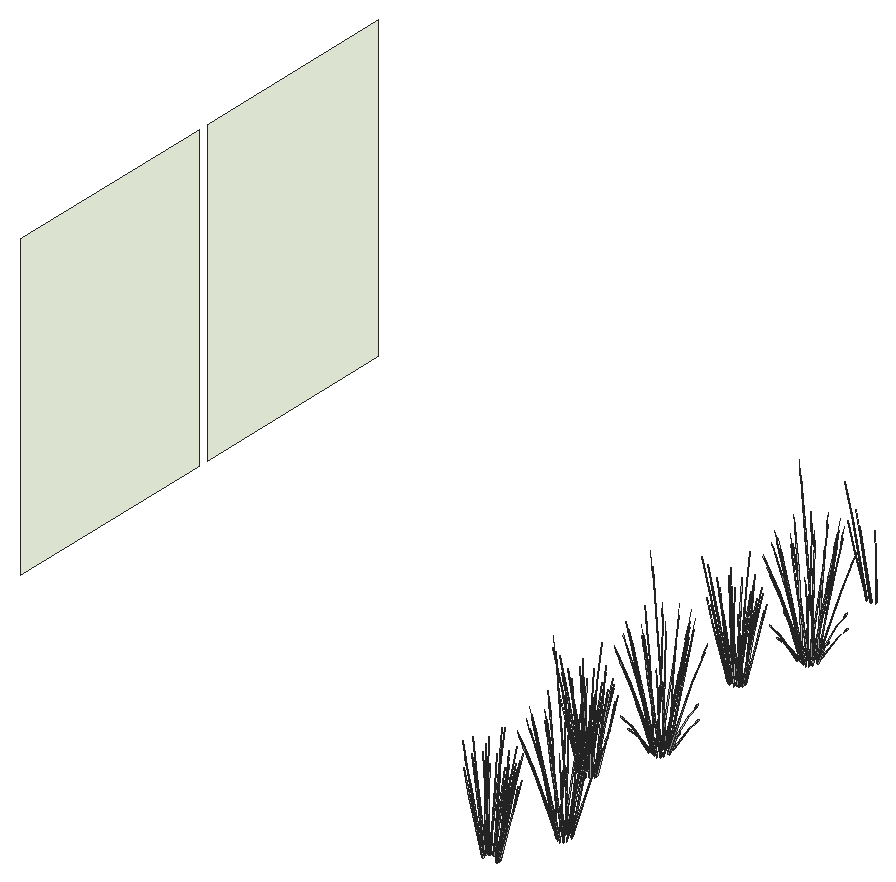
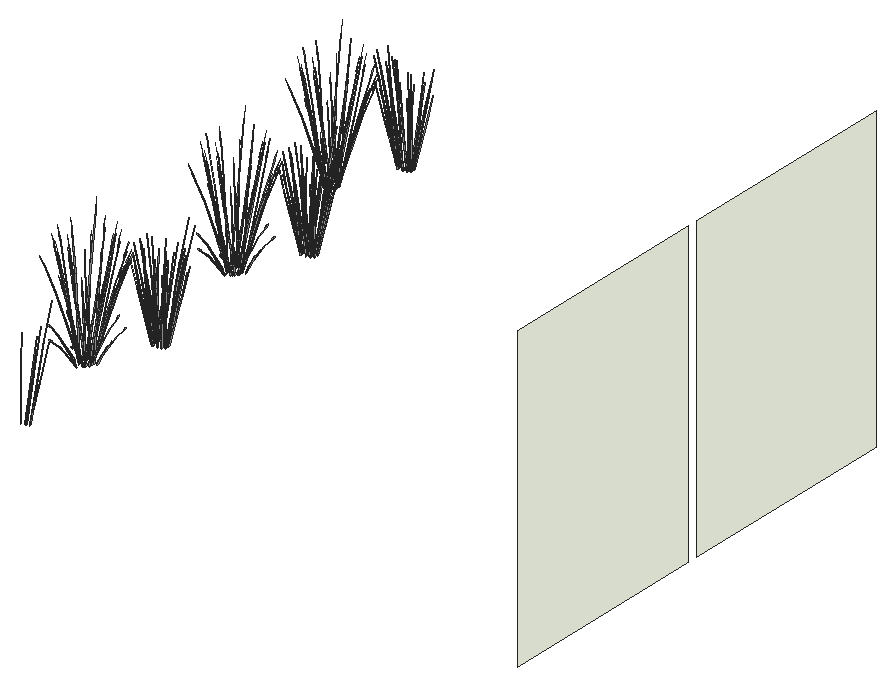
# SketchUp Ruby script. Lengths in inches.
U = 1.inch
M = Sketchup.active_model
def pt(a) = Geom::Point3d.new(a.map { |v| v * U })
def face(e, loops, mat)
  f = e.add_face(loops[0].map { |a| pt(a) })
  loops[1..].each { |l| e.add_face(l.map { |a| pt(a) }).erase! }
  f.material = f.back_material = mat if mat
  f
end
# faces: each face lists its corners as indices into pts; further lists are holes
def faces(e, pts, list, mat = nil) = list.each { |f| face(e, (f[0].is_a?(Array) ? f : [f]).map { |l| l.map { |i| pts[i] } }, mat) }
# xy, xz, yz: faces in a plane at the given z, y or x. An outline is a flat list of corners, or four numbers for a rectangle; further outlines are holes
def ring(l) = l.size == 4 ? [[l[0], l[1]], [l[2], l[1]], [l[2], l[3]], [l[0], l[3]]] : l.each_slice(2).to_a
def flat(e, list, mat, &to3) = list.each { |f| face(e, (f[0].is_a?(Array) ? f : [f]).map { |l| ring(l).map { |u, v| to3.(u, v) } }, mat) }
def xy(e, z, list, mat = nil) = flat(e, list, mat) { |x, y| [x, y, z] }
def xz(e, y, list, mat = nil) = flat(e, list, mat) { |x, z| [x, y, z] }
def yz(e, x, list, mat = nil) = flat(e, list, mat) { |y, z| [x, y, z] }
def lines(e, pts, list) = list.each { |a, b| e.add_line(pt(pts[a]), pt(pts[b])) }
# prism: a flat outline (further loops are holes) pulled along v
def prism(e, loops, v, mat = nil)
  f = face(e, loops, mat); d = Geom::Vector3d.new(v.map { |x| x * U })
  f.pushpull(f.normal.samedirection?(d) ? d.length : -d.length)
end
def box(e, o, s, mat = nil) = prism(e, [[o, [o[0] + s[0], o[1], o[2]], [o[0] + s[0], o[1] + s[1], o[2]], [o[0], o[1] + s[1], o[2]]]], [0, 0, s[2]], mat)
def at(x, y, z, deg = 0) = Geom::Transformation.translation(pt([x, y, z])) * Geom::Transformation.rotation(ORIGIN, Z_AXIS, deg.degrees)
def axes(o, x, y, z) = Geom::Transformation.new([*x, 0, *y, 0, *z, 0, *pt(o).to_a, 1])
def part(name) = M.definitions.add(name)
# library, detail: a bought-in or finely detailed component or shape, given as its bounding box
def library(name, o, s) = part(name).tap { |d| box(d.entities, o, s) }
def detail(e, o, s) = box(e.add_group.entities, o, s)
def put(e, d, t, mat = nil) = e.add_instance(d, t).tap { |i| i.material = mat if mat }
def group(e, t, mat = nil) = e.add_group.tap { |g| g.transformation = t; g.material = mat if mat }.entities
root = M.entities
M.materials.add("Glass_Basic_1").color = [156, 186, 90]
M.materials["Glass_Basic_1"].alpha = 0.25
M.materials.add("LightPink_Translucent").color = [175, 214, 192]
M.materials["LightPink_Translucent"].alpha = 0.75
c1 = part("blade")
p = [[2.15,0.21,22],[0,0.17,0],[0.09,0.45,0],[2.18,0.31,22],[2.29,0.31,22],[0.38,0.45,0],
  [2.48,0.24,33],[2.49,0.24,33],[2.48,0.22,33]]
faces(c1.entities,p,[[0,1,2,3],[4,5,2,3],[6,3,4,7],[8,0,3,6]])
c2 = part("blade with seeds\#1")
put(c2.entities,c1,at(0,0,0))
c3 = part("seeds")
p = [[0.3,-0.1,1.38],[-0.01,-0.03,1.59],[-0.01,-0.03,0.03],[0.14,-0.07,-0.07],[0.29,-0.03,3],[0.15,0.01,3.11]]
faces(c3.entities,p,[[0,1,2,3],[1,0,4,5]],"LightPink_Translucent")
c4 = part("blade with seeds")
put(c4.entities,c1,at(0,0,0))
put(c4.entities,c3,axes([2.4,0.25,30.99],[1.5799,-0.05474,1.17369],[-0.12525,1.92788,0.29478],[-0.07173,-0.02425,1.56792]))
yz(root,330,[[388.5,141,453,228],[456,141,517.5,228]],"Glass_Basic_1")
put(root,c2,axes([495.49,353.2,140.96],[-0.43273,0.05446,0.29052],[-0.11427,-0.31131,-0.37506],[0.12401,-0.08362,0.71765]))
put(root,c2,axes([495.79,353.08,140.7],[0.12329,0.35069,0.39379],[-0.48364,0.06086,0.3247],[0.14254,-0.08248,0.81485]))
put(root,c2,axes([495.88,353.15,140.69],[0.34128,0.16025,0.05275],[-0.1987,0.22821,0.41527],[0.10942,-0.07378,0.63322]))
put(root,c2,axes([492.04,352.71,140.96],[0.28286,0.23857,0.29052],[-0.32298,0.22584,-0.37506],[-0.1641,-0.03436,0.71765]))
put(root,c2,axes([495.56,353.94,140.96],[-0.41315,-0.1063,0.29052],[0.1205,-0.31012,-0.37506],[0.16634,-0.02844,0.71765]))
put(root,c2,axes([491.24,353.375,140.7],[0.14045,-0.34743,0.39379],[0.46175,0.1188,0.3247],[-0.18159,0.02088,0.81485]))
put(root,c2,axes([491.2,353.28,140.69],[-0.18259,-0.25981,0.05275],[0.33295,-0.12717,0.41527],[-0.14677,0.02509,0.63322]))
put(root,c2,axes([495.93,354.04,140.69],[0.18259,0.25981,0.05275],[-0.33295,0.12717,0.41527],[0.14677,-0.02509,0.63322]))
put(root,c2,axes([495.9,353.94,140.7],[-0.14045,0.34743,0.39379],[-0.46175,-0.1188,0.3247],[0.18159,-0.02088,0.81485]))
put(root,c2,axes([491.57,353.38,140.96],[0.41315,0.1063,0.29052],[-0.1205,0.31012,-0.37506],[-0.16634,0.02844,0.71765]))
put(root,c2,axes([495.1,354.61,140.96],[-0.28286,-0.23857,0.29052],[0.32298,-0.22584,-0.37506],[0.1641,0.03436,0.71765]))
put(root,c2,axes([491.25,354.17,140.69],[-0.34128,-0.16025,0.05275],[0.1987,-0.22821,0.41527],[-0.10942,0.07378,0.63322]))
put(root,c2,axes([491.35,354.24,140.7],[-0.12329,-0.35069,0.39379],[0.48364,-0.06086,0.3247],[-0.14254,0.08248,0.81485]))
put(root,c2,axes([491.64,354.12,140.96],[0.43273,-0.05446,0.29052],[0.11427,0.31131,-0.37506],[-0.12401,0.08362,0.71765]))
put(root,c2,axes([495.35,354.83,140.69],[-0.02503,0.28975,0.05275],[-0.378,-0.00794,0.41527],[0.1448,0.03032,0.63322]))
put(root,c2,axes([495.39,354.73,140.7],[-0.36656,0.25108,0.39379],[-0.31614,-0.26664,0.3247],[0.17198,0.04631,0.81485]))
put(root,c2,axes([490.66,355.01,141.44],[0.43869,0.10171,-0.05322],[-0.13494,0.31305,-0.24131],[-0.07175,0.04753,0.79594]))
put(root,c2,axes([494.22,355.02,140.96],[-0.07678,-0.30692,0.29052],[0.43892,-0.08104,-0.37506],[0.11789,0.08795,0.71765]))
put(root,c2,axes([492.23,354.74,140.96],[0.33637,-0.20062,0.29052],[0.31842,0.22908,-0.37506],[-0.04845,0.11639,0.71765]))
put(root,c2,axes([491.92,354.92,140.69],[-0.40853,-0.01775,0.05275],[0.0112,-0.2681,0.41527],[-0.04275,0.1027,0.63322]))
put(root,c2,axes([492.05,354.95,140.7],[-0.354,-0.25999,0.39379],[0.37594,-0.22422,0.3247],[-0.0653,0.12198,0.81485]))
put(root,c2,axes([493.17,355.07,140.96],[0.14987,-0.29303,0.29052],[0.43725,0.08547,-0.37506],[0.04009,0.11798,0.71765]))
put(root,c2,axes([494.29,355.3,140.69],[-0.22594,0.24206,0.05275],[-0.32175,-0.14093,0.41527],[0.10402,0.07761,0.63322]))
put(root,c2,axes([494.39,355.23,140.7],[-0.49445,0.08745,0.39379],[-0.08581,-0.34303,0.3247],[0.11629,0.1011,0.81485]))
put(root,c2,axes([493.76,356.12,141.44],[0.34354,-0.2186,-0.05322],[0.31478,0.23941,-0.24131],[0.02216,0.06784,0.79594]))
put(root,c2,axes([493.04,355.34,140.69],[-0.36632,0.1295,0.05275],[-0.1793,-0.23615,0.41527],[0.03538,0.1041,0.63322]))
put(root,c2,axes([492.01,354.8,141.24],[0.54637,0.01888,-0.11073],[-0.01493,0.35746,-0.6146],[-0.03795,0.13767,0.93387]))
put(root,c2,axes([493.17,355.3125,140.97],[-0.48986,-0.09962,0.43711],[0.16751,-0.3275,0.36041],[0.02944,0.12879,0.90448]))
put(root,c4,axes([501.13,369.24,140.79],[0.01009,0.19824,1.55952],[-0.43714,-0.13151,0.1261],[0.02704,-0.28251,0.66668]))
put(root,c4,axes([500.36,369.32,140.79],[0.0942,0.16583,1.55952],[-0.43527,0.13961,0.1261],[-0.09838,-0.26034,0.66668]))
put(root,c4,axes([501.83,369.61,140.79],[-0.07673,0.17753,1.55952],[-0.32188,-0.36739,0.1261],[0.14521,-0.22898,0.66668]))
put(root,c4,axes([500.92,369.3125,141.85],[-0.40325,0.24047,-0.11066],[-0.19816,-0.4268,-0.6142],[-0.0532,-0.17986,0.93327]))
put(root,c4,axes([501.75,369.85,141.85],[-0.45289,-0.02559,-0.11066],[0.01238,-0.48454,-0.6142],[0.03146,-0.18661,0.93327]))
put(root,c4,axes([500.07,369.92,140.79],[0.13683,0.11937,1.55952],[-0.36934,0.30141,0.1261],[-0.1682,-0.20674,0.66668]))
put(root,c4,axes([499.73,369.83,140.79],[0.15307,0.08899,1.55952],[-0.31677,0.37333,0.1261],[-0.19743,-0.16841,0.66668]))
put(root,c4,axes([499.96,369.33,141.85],[-0.24556,0.44211,-0.11066],[-0.35561,-0.2547,-0.6142],[-0.12361,-0.12491,0.93327]))
put(root,c4,axes([502.28,370.34,140.79],[-0.14298,0.10925,1.55952],[-0.12037,-0.50484,0.1261],[0.22447,-0.1141,0.66668]))
put(root,c4,axes([502.26,371.92,141.85],[-0.20734,-0.4677,-0.11066],[0.36799,-0.22984,-0.6142],[0.15507,-0.06171,0.93327]))
put(root,c4,axes([499.41,370.65,140.79],[0.17092,-0.0117,1.55952],[-0.11339,0.50701,0.1261],[-0.24358,-0.03136,0.66668]))
put(root,c4,axes([498.67,370.87,141.85],[0.20734,0.4677,-0.11066],[-0.36799,0.22984,-0.6142],[-0.15507,0.06171,0.93327]))
put(root,c4,axes([501.8,372.89,141.85],[0.02206,-0.52527,-0.11066],[0.41777,0.01436,-0.6142],[0.1609,0.03649,0.93327]))
put(root,c4,axes([499.48,371.54,140.79],[0.14298,-0.10925,1.55952],[0.12037,0.50484,0.1261],[-0.22447,0.1141,0.66668]))
put(root,c4,axes([500.93,372.31,141.34],[0.23139,-0.41299,1.25837],[0.36026,0.43608,0.54295],[-0.21711,0.13325,1.21634]))
put(root,c4,axes([502.03,372.05,140.79],[-0.15307,-0.08899,1.55952],[0.31677,-0.37333,0.1261],[0.19743,0.16841,0.66668]))
put(root,c4,axes([498.68,371.98,141.85],[0.38119,0.2848,-0.11066],[-0.21961,0.41244,-0.6142],[-0.10769,0.14337,0.93327]))
put(root,c4,axes([500.97,373.46,141.85],[0.24556,-0.44211,-0.11066],[0.35561,0.2547,-0.6142],[0.12361,0.12491,0.93327]))
put(root,c4,axes([499.17,374.06,140.84],[0.37435,-0.09148,-0.03177],[0.08606,0.43236,-0.14407],[-0.02373,0.09029,0.47519]))
put(root,c4,axes([499.92,372.27,140.79],[0.07673,-0.17753,1.55952],[0.32188,0.36739,0.1261],[-0.14521,0.22898,0.66668]))
put(root,c4,axes([499.18,372.9375,141.85],[0.45289,0.02559,-0.11066],[-0.01238,0.48454,-0.6142],[-0.03146,0.18661,0.93327]))
put(root,c4,axes([500.02,373.48,141.85],[0.40325,-0.24047,-0.11066],[0.19816,0.4268,-0.6142],[0.0532,0.17986,0.93327]))
put(root,c4,axes([500.625,372.65,140.79],[-0.01009,-0.19824,1.55952],[0.43714,0.13151,0.1261],[-0.02704,0.28251,0.66668]))
put(root,c2,axes([485.28,396.15,140.9],[0.55379,-0.09794,0.44104],[0.09611,0.38419,0.36366],[-0.13024,-0.11323,0.91263]))
put(root,c2,axes([486.66,396.19,140.6],[0.36632,-0.1295,0.05275],[0.1793,0.23615,0.41527],[-0.03538,-0.1041,0.63322]))
put(root,c2,axes([485.4,396.23,140.6],[0.22594,-0.24206,0.05275],[0.32175,0.14093,0.41527],[-0.10402,-0.07761,0.63322]))
put(root,c2,axes([486.52,396.46,140.86],[-0.14987,0.29303,0.29052],[-0.43725,-0.08547,-0.37506],[-0.04009,-0.11798,0.71765]))
put(root,c2,axes([487.77,396.61,140.6],[0.40853,0.01775,0.05275],[-0.0112,0.2681,0.41527],[0.04275,-0.1027,0.63322]))
put(root,c2,axes([487.46,396.79,140.86],[-0.33637,0.20062,0.29052],[-0.31842,-0.22908,-0.37506],[0.04845,-0.11639,0.71765]))
put(root,c2,axes([485.47,396.51,140.86],[0.07678,0.30692,0.29052],[-0.43892,0.08104,-0.37506],[-0.11789,-0.08795,0.71765]))
put(root,c2,axes([484.15,396.71,140.9],[0.41055,-0.28121,0.44104],[0.35407,0.29863,0.36366],[-0.19262,-0.05187,0.91263]))
put(root,c2,axes([484.34,396.71,140.6],[0.02503,-0.28975,0.05275],[0.378,0.00794,0.41527],[-0.1448,-0.03032,0.63322]))
put(root,c2,axes([488.05,397.41,140.86],[-0.43273,0.05446,0.29052],[-0.11427,-0.31131,-0.37506],[0.12401,-0.08362,0.71765]))
put(root,c2,axes([488.44,397.36,140.6],[0.34128,0.16025,0.05275],[-0.1987,0.22821,0.41527],[0.10942,-0.07378,0.63322]))
put(root,c2,axes([484.6,396.92,140.86],[0.28286,0.23857,0.29052],[-0.32298,0.22584,-0.37506],[-0.1641,-0.03436,0.71765]))
put(root,c2,axes([488.12,398.15,140.86],[-0.41315,-0.1063,0.29052],[0.1205,-0.31012,-0.37506],[0.16634,-0.02844,0.71765]))
put(root,c2,axes([483.76,397.49,140.6],[-0.18259,-0.25981,0.05275],[0.33295,-0.12717,0.41527],[-0.14677,0.02509,0.63322]))
put(root,c2,axes([488.49,398.25,140.6],[0.18259,0.25981,0.05275],[-0.33295,0.12717,0.41527],[0.14677,-0.02509,0.63322]))
put(root,c2,axes([484.13,397.59,140.86],[0.41315,0.1063,0.29052],[-0.1205,0.31012,-0.37506],[-0.16634,0.02844,0.71765]))
put(root,c2,axes([487.65,398.82,140.86],[-0.28286,-0.23857,0.29052],[0.32298,-0.22584,-0.37506],[0.1641,0.03436,0.71765]))
put(root,c2,axes([483.81,398.38,140.6],[-0.34128,-0.16025,0.05275],[0.1987,-0.22821,0.41527],[-0.10942,0.07378,0.63322]))
put(root,c2,axes([484.2,398.34,140.86],[0.43273,-0.05446,0.29052],[0.11427,0.31131,-0.37506],[-0.12401,0.08362,0.71765]))
put(root,c2,axes([487.91,399.04,140.6],[-0.02503,0.28975,0.05275],[-0.378,-0.00794,0.41527],[0.1448,0.03032,0.63322]))
put(root,c2,axes([483.22,399.22,141.35],[0.43869,0.10171,-0.05322],[-0.13494,0.31305,-0.24131],[-0.07175,0.04753,0.79594]))
put(root,c2,axes([486.78,399.24,140.86],[-0.07678,-0.30692,0.29052],[0.43892,-0.08104,-0.37506],[0.11789,0.08795,0.71765]))
put(root,c2,axes([484.79,398.96,140.86],[0.33637,-0.20062,0.29052],[0.31842,0.22908,-0.37506],[-0.04845,0.11639,0.71765]))
put(root,c2,axes([484.48,399.14,140.6],[-0.40853,-0.01775,0.05275],[0.0112,-0.2681,0.41527],[-0.04275,0.1027,0.63322]))
put(root,c2,axes([485.73,399.29,140.86],[0.14987,-0.29303,0.29052],[0.43725,0.08547,-0.37506],[0.04009,0.11798,0.71765]))
put(root,c2,axes([486.85,399.52,140.6],[-0.22594,0.24206,0.05275],[-0.32175,-0.14093,0.41527],[0.10402,0.07761,0.63322]))
put(root,c2,axes([486.32,400.33,141.35],[0.34354,-0.2186,-0.05322],[0.31478,0.23941,-0.24131],[0.02216,0.06784,0.79594]))
put(root,c2,axes([485.59,399.55,140.6],[-0.36632,0.1295,0.05275],[-0.1793,-0.23615,0.41527],[0.03538,0.1041,0.63322]))
put(root,c2,axes([485.72,399.53,140.87],[-0.48986,-0.09962,0.43711],[0.16751,-0.3275,0.36041],[0.02944,0.12879,0.90448]))
put(root,c4,axes([493.6875,413.45,140.7],[0.01009,0.19824,1.55952],[-0.43714,-0.13151,0.1261],[0.02704,-0.28251,0.66668]))
put(root,c4,axes([492.92,413.53,140.7],[0.0942,0.16583,1.55952],[-0.43527,0.13961,0.1261],[-0.09838,-0.26034,0.66668]))
put(root,c4,axes([493.07,413.02,141.46],[-0.05782,-0.07805,1.59199],[-0.42244,0.00664,-0.25177],[-0.05494,-0.1789,0.12768]))
put(root,c4,axes([494.39,413.82,140.7],[-0.07673,0.17753,1.55952],[-0.32188,-0.36739,0.1261],[0.14521,-0.22898,0.66668]))
put(root,c4,axes([495.1,413.79,141.46],[0.00314,-0.10283,1.59199],[-0.31434,-0.32739,-0.25177],[0.06423,-0.17468,0.12768]))
put(root,c4,axes([493.47,413.52,141.75],[-0.40325,0.24047,-0.11066],[-0.19816,-0.4268,-0.6142],[-0.0532,-0.17986,0.93327]))
put(root,c4,axes([494.3125,414.07,141.75],[-0.45289,-0.02559,-0.11066],[0.01238,-0.48454,-0.6142],[0.03146,-0.18661,0.93327]))
put(root,c4,axes([492.625,414.14,140.7],[0.13683,0.11937,1.55952],[-0.36934,0.30141,0.1261],[-0.1682,-0.20674,0.66668]))
put(root,c4,axes([492.29,414.05,140.7],[0.15307,0.08899,1.55952],[-0.31677,0.37333,0.1261],[-0.19743,-0.16841,0.66668]))
put(root,c4,axes([491.49,413.04,141.46],[-0.08813,-0.01188,1.59199],[-0.30658,0.33715,-0.25177],[-0.14498,-0.08826,0.12768]))
put(root,c4,axes([492.51,413.54,141.75],[-0.24556,0.44211,-0.11066],[-0.35561,-0.2547,-0.6142],[-0.12361,-0.12491,0.93327]))
put(root,c4,axes([494.83,414.55,140.7],[-0.14298,0.10925,1.55952],[-0.12037,-0.50484,0.1261],[0.22447,-0.1141,0.66668]))
put(root,c4,axes([495.78,415.39,141.46],[0.06244,-0.0731,1.59199],[-0.03959,-0.48785,-0.25177],[0.14934,-0.07786,0.12768]))
put(root,c4,axes([494.82,416.13,141.75],[-0.20734,-0.4677,-0.11066],[0.36799,-0.22984,-0.6142],[0.15507,-0.06171,0.93327]))
put(root,c4,axes([491.96,414.86,140.7],[0.17092,-0.0117,1.55952],[-0.11339,0.50701,0.1261],[-0.24358,-0.03136,0.66668]))
put(root,c4,axes([490.4,414.98,141.46],[-0.07171,0.06058,1.59199],[-0.02817,0.48891,-0.25177],[-0.15815,0.04916,0.12768]))
put(root,c4,axes([491.23,415.09,141.75],[0.20734,0.4677,-0.11066],[-0.36799,0.22984,-0.6142],[-0.15507,0.06171,0.93327]))
put(root,c4,axes([494.35,417.1,141.75],[0.02206,-0.52527,-0.11066],[0.41777,0.01436,-0.6142],[0.1609,0.03649,0.93327]))
put(root,c4,axes([492.04,415.75,140.7],[0.14298,-0.10925,1.55952],[0.12037,0.50484,0.1261],[-0.22447,0.1141,0.66668]))
put(root,c4,axes([493.49,416.52,141.24],[0.23139,-0.41299,1.25837],[0.36026,0.43608,0.54295],[-0.21711,0.13325,1.21634]))
put(root,c4,axes([495.02,417.58,141.46],[0.08863,-0.00461,1.59199],[0.25616,-0.38966,-0.25177],[0.15528,0.06024,0.12768]))
put(root,c4,axes([494.58,416.26,140.7],[-0.15307,-0.08899,1.55952],[0.31677,-0.37333,0.1261],[0.19743,0.16841,0.66668]))
put(root,c4,axes([491.24,416.2,141.75],[0.38119,0.2848,-0.11066],[-0.21961,0.41244,-0.6142],[-0.10769,0.14337,0.93327]))
put(root,c4,axes([493.53,417.67,141.75],[0.24556,-0.44211,-0.11066],[0.35561,0.2547,-0.6142],[0.12361,0.12491,0.93327]))
put(root,c4,axes([492.48,416.49,140.7],[0.07673,-0.17753,1.55952],[0.32188,0.36739,0.1261],[-0.14521,0.22898,0.66668]))
put(root,c4,axes([491.73,417.15,141.75],[0.45289,0.02559,-0.11066],[-0.01238,0.48454,-0.6142],[-0.03146,0.18661,0.93327]))
put(root,c4,axes([492.57,417.69,141.75],[0.40325,-0.24047,-0.11066],[0.19816,0.4268,-0.6142],[0.0532,0.17986,0.93327]))
put(root,c4,axes([492.01,417.57,141.46],[0.00753,0.10253,1.59199],[0.34598,0.28122,-0.25177],[-0.04567,0.18237,0.12768]))
put(root,c4,axes([493.18,416.86,140.7],[-0.01009,-0.19824,1.55952],[0.43714,0.13151,0.1261],[-0.02704,0.28251,0.66668]))
put(root,c4,axes([493.2,419,141.46],[0.06783,0.06632,1.59199],[0.4161,-0.08489,-0.25177],[0.07889,0.16641,0.12768]))
put(root,c2,axes([485.28,449.72,140.9],[0.55379,-0.09794,0.44104],[0.09611,0.38419,0.36366],[-0.13024,-0.11323,0.91263]))
put(root,c2,axes([486.66,449.77,140.6],[0.36632,-0.1295,0.05275],[0.1793,0.23615,0.41527],[-0.03538,-0.1041,0.63322]))
put(root,c2,axes([485.4,449.8,140.6],[0.22594,-0.24206,0.05275],[0.32175,0.14093,0.41527],[-0.10402,-0.07761,0.63322]))
put(root,c2,axes([486.52,450.03,140.86],[-0.14987,0.29303,0.29052],[-0.43725,-0.08547,-0.37506],[-0.04009,-0.11798,0.71765]))
put(root,c2,axes([487.77,450.18,140.6],[0.40853,0.01775,0.05275],[-0.0112,0.2681,0.41527],[0.04275,-0.1027,0.63322]))
put(root,c2,axes([487.46,450.36,140.86],[-0.33637,0.20062,0.29052],[-0.31842,-0.22908,-0.37506],[0.04845,-0.11639,0.71765]))
put(root,c2,axes([485.47,450.08,140.86],[0.07678,0.30692,0.29052],[-0.43892,0.08104,-0.37506],[-0.11789,-0.08795,0.71765]))
put(root,c2,axes([484.15,450.28,140.9],[0.41055,-0.28121,0.44104],[0.35407,0.29863,0.36366],[-0.19262,-0.05187,0.91263]))
put(root,c2,axes([484.34,450.28,140.6],[0.02503,-0.28975,0.05275],[0.378,0.00794,0.41527],[-0.1448,-0.03032,0.63322]))
put(root,c2,axes([488.05,450.98,140.86],[-0.43273,0.05446,0.29052],[-0.11427,-0.31131,-0.37506],[0.12401,-0.08362,0.71765]))
put(root,c2,axes([488.44,450.93,140.6],[0.34128,0.16025,0.05275],[-0.1987,0.22821,0.41527],[0.10942,-0.07378,0.63322]))
put(root,c2,axes([484.6,450.5,140.86],[0.28286,0.23857,0.29052],[-0.32298,0.22584,-0.37506],[-0.1641,-0.03436,0.71765]))
put(root,c2,axes([488.12,451.73,140.86],[-0.41315,-0.1063,0.29052],[0.1205,-0.31012,-0.37506],[0.16634,-0.02844,0.71765]))
put(root,c2,axes([483.76,451.07,140.6],[-0.18259,-0.25981,0.05275],[0.33295,-0.12717,0.41527],[-0.14677,0.02509,0.63322]))
put(root,c2,axes([488.49,451.82,140.6],[0.18259,0.25981,0.05275],[-0.33295,0.12717,0.41527],[0.14677,-0.02509,0.63322]))
put(root,c2,axes([484.13,451.16,140.86],[0.41315,0.1063,0.29052],[-0.1205,0.31012,-0.37506],[-0.16634,0.02844,0.71765]))
put(root,c2,axes([487.65,452.4,140.86],[-0.28286,-0.23857,0.29052],[0.32298,-0.22584,-0.37506],[0.1641,0.03436,0.71765]))
put(root,c2,axes([483.81,451.96,140.6],[-0.34128,-0.16025,0.05275],[0.1987,-0.22821,0.41527],[-0.10942,0.07378,0.63322]))
put(root,c2,axes([484.2,451.91,140.86],[0.43273,-0.05446,0.29052],[0.11427,0.31131,-0.37506],[-0.12401,0.08362,0.71765]))
put(root,c2,axes([487.91,452.61,140.6],[-0.02503,0.28975,0.05275],[-0.378,-0.00794,0.41527],[0.1448,0.03032,0.63322]))
put(root,c2,axes([483.22,452.79,141.35],[0.43869,0.10171,-0.05322],[-0.13494,0.31305,-0.24131],[-0.07175,0.04753,0.79594]))
put(root,c2,axes([486.78,452.8125,140.86],[-0.07678,-0.30692,0.29052],[0.43892,-0.08104,-0.37506],[0.11789,0.08795,0.71765]))
put(root,c2,axes([484.79,452.53,140.86],[0.33637,-0.20062,0.29052],[0.31842,0.22908,-0.37506],[-0.04845,0.11639,0.71765]))
put(root,c2,axes([484.48,452.71,140.6],[-0.40853,-0.01775,0.05275],[0.0112,-0.2681,0.41527],[-0.04275,0.1027,0.63322]))
put(root,c2,axes([485.73,452.86,140.86],[0.14987,-0.29303,0.29052],[0.43725,0.08547,-0.37506],[0.04009,0.11798,0.71765]))
put(root,c2,axes([486.85,453.09,140.6],[-0.22594,0.24206,0.05275],[-0.32175,-0.14093,0.41527],[0.10402,0.07761,0.63322]))
put(root,c2,axes([486.32,453.9,141.35],[0.34354,-0.2186,-0.05322],[0.31478,0.23941,-0.24131],[0.02216,0.06784,0.79594]))
put(root,c2,axes([485.59,453.125,140.6],[-0.36632,0.1295,0.05275],[-0.1793,-0.23615,0.41527],[0.03538,0.1041,0.63322]))
put(root,c2,axes([485.72,453.1,140.87],[-0.48986,-0.09962,0.43711],[0.16751,-0.3275,0.36041],[0.02944,0.12879,0.90448]))
put(root,c4,axes([493.6875,467.02,140.7],[0.01009,0.19824,1.55952],[-0.43714,-0.13151,0.1261],[0.02704,-0.28251,0.66668]))
put(root,c4,axes([492.92,467.1,140.7],[0.0942,0.16583,1.55952],[-0.43527,0.13961,0.1261],[-0.09838,-0.26034,0.66668]))
put(root,c4,axes([493.07,466.6,141.46],[-0.05782,-0.07805,1.59199],[-0.42244,0.00664,-0.25177],[-0.05494,-0.1789,0.12768]))
put(root,c4,axes([494.39,467.4,140.7],[-0.07673,0.17753,1.55952],[-0.32188,-0.36739,0.1261],[0.14521,-0.22898,0.66668]))
put(root,c4,axes([495.1,467.36,141.46],[0.00314,-0.10283,1.59199],[-0.31434,-0.32739,-0.25177],[0.06423,-0.17468,0.12768]))
put(root,c4,axes([493.47,467.1,141.75],[-0.40325,0.24047,-0.11066],[-0.19816,-0.4268,-0.6142],[-0.0532,-0.17986,0.93327]))
put(root,c4,axes([494.3125,467.64,141.75],[-0.45289,-0.02559,-0.11066],[0.01238,-0.48454,-0.6142],[0.03146,-0.18661,0.93327]))
put(root,c4,axes([492.625,467.71,140.7],[0.13683,0.11937,1.55952],[-0.36934,0.30141,0.1261],[-0.1682,-0.20674,0.66668]))
put(root,c4,axes([492.29,467.62,140.7],[0.15307,0.08899,1.55952],[-0.31677,0.37333,0.1261],[-0.19743,-0.16841,0.66668]))
put(root,c4,axes([491.49,466.61,141.46],[-0.08813,-0.01188,1.59199],[-0.30658,0.33715,-0.25177],[-0.14498,-0.08826,0.12768]))
put(root,c4,axes([492.51,467.12,141.75],[-0.24556,0.44211,-0.11066],[-0.35561,-0.2547,-0.6142],[-0.12361,-0.12491,0.93327]))
put(root,c4,axes([494.83,468.13,140.7],[-0.14298,0.10925,1.55952],[-0.12037,-0.50484,0.1261],[0.22447,-0.1141,0.66668]))
put(root,c4,axes([495.78,468.96,141.46],[0.06244,-0.0731,1.59199],[-0.03959,-0.48785,-0.25177],[0.14934,-0.07786,0.12768]))
put(root,c4,axes([494.82,469.7,141.75],[-0.20734,-0.4677,-0.11066],[0.36799,-0.22984,-0.6142],[0.15507,-0.06171,0.93327]))
put(root,c4,axes([491.96,468.44,140.7],[0.17092,-0.0117,1.55952],[-0.11339,0.50701,0.1261],[-0.24358,-0.03136,0.66668]))
put(root,c4,axes([490.4,468.55,141.46],[-0.07171,0.06058,1.59199],[-0.02817,0.48891,-0.25177],[-0.15815,0.04916,0.12768]))
put(root,c4,axes([491.23,468.66,141.75],[0.20734,0.4677,-0.11066],[-0.36799,0.22984,-0.6142],[-0.15507,0.06171,0.93327]))
put(root,c4,axes([494.35,470.68,141.75],[0.02206,-0.52527,-0.11066],[0.41777,0.01436,-0.6142],[0.1609,0.03649,0.93327]))
put(root,c4,axes([492.04,469.33,140.7],[0.14298,-0.10925,1.55952],[0.12037,0.50484,0.1261],[-0.22447,0.1141,0.66668]))
put(root,c4,axes([493.49,470.09,141.24],[0.23139,-0.41299,1.25837],[0.36026,0.43608,0.54295],[-0.21711,0.13325,1.21634]))
put(root,c4,axes([495.02,471.15,141.46],[0.08863,-0.00461,1.59199],[0.25616,-0.38966,-0.25177],[0.15528,0.06024,0.12768]))
put(root,c4,axes([494.58,469.83,140.7],[-0.15307,-0.08899,1.55952],[0.31677,-0.37333,0.1261],[0.19743,0.16841,0.66668]))
put(root,c4,axes([491.24,469.77,141.75],[0.38119,0.2848,-0.11066],[-0.21961,0.41244,-0.6142],[-0.10769,0.14337,0.93327]))
put(root,c4,axes([493.53,471.25,141.75],[0.24556,-0.44211,-0.11066],[0.35561,0.2547,-0.6142],[0.12361,0.12491,0.93327]))
put(root,c4,axes([492.48,470.06,140.7],[0.07673,-0.17753,1.55952],[0.32188,0.36739,0.1261],[-0.14521,0.22898,0.66668]))
put(root,c4,axes([491.73,470.72,141.75],[0.45289,0.02559,-0.11066],[-0.01238,0.48454,-0.6142],[-0.03146,0.18661,0.93327]))
put(root,c4,axes([492.57,471.26,141.75],[0.40325,-0.24047,-0.11066],[0.19816,0.4268,-0.6142],[0.0532,0.17986,0.93327]))
put(root,c4,axes([492.01,471.15,141.46],[0.00753,0.10253,1.59199],[0.34598,0.28122,-0.25177],[-0.04567,0.18237,0.12768]))
put(root,c4,axes([493.18,470.43,140.7],[-0.01009,-0.19824,1.55952],[0.43714,0.13151,0.1261],[-0.02704,0.28251,0.66668]))
put(root,c4,axes([493.2,472.57,141.46],[0.06783,0.06632,1.59199],[0.4161,-0.08489,-0.25177],[0.07889,0.16641,0.12768]))
put(root,c2,axes([485.28,498.93,140.9],[0.55379,-0.09794,0.44104],[0.09611,0.38419,0.36366],[-0.13024,-0.11323,0.91263]))
put(root,c2,axes([486.66,498.98,140.6],[0.36632,-0.1295,0.05275],[0.1793,0.23615,0.41527],[-0.03538,-0.1041,0.63322]))
put(root,c2,axes([485.4,499.01,140.6],[0.22594,-0.24206,0.05275],[0.32175,0.14093,0.41527],[-0.10402,-0.07761,0.63322]))
put(root,c2,axes([486.52,499.24,140.86],[-0.14987,0.29303,0.29052],[-0.43725,-0.08547,-0.37506],[-0.04009,-0.11798,0.71765]))
put(root,c2,axes([487.77,499.39,140.6],[0.40853,0.01775,0.05275],[-0.0112,0.2681,0.41527],[0.04275,-0.1027,0.63322]))
